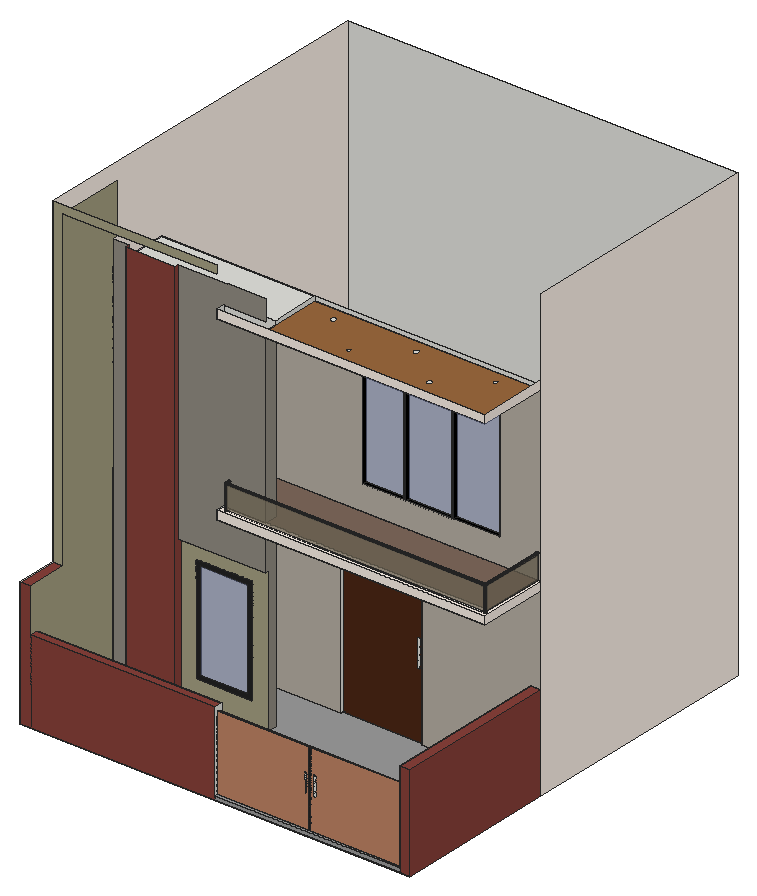
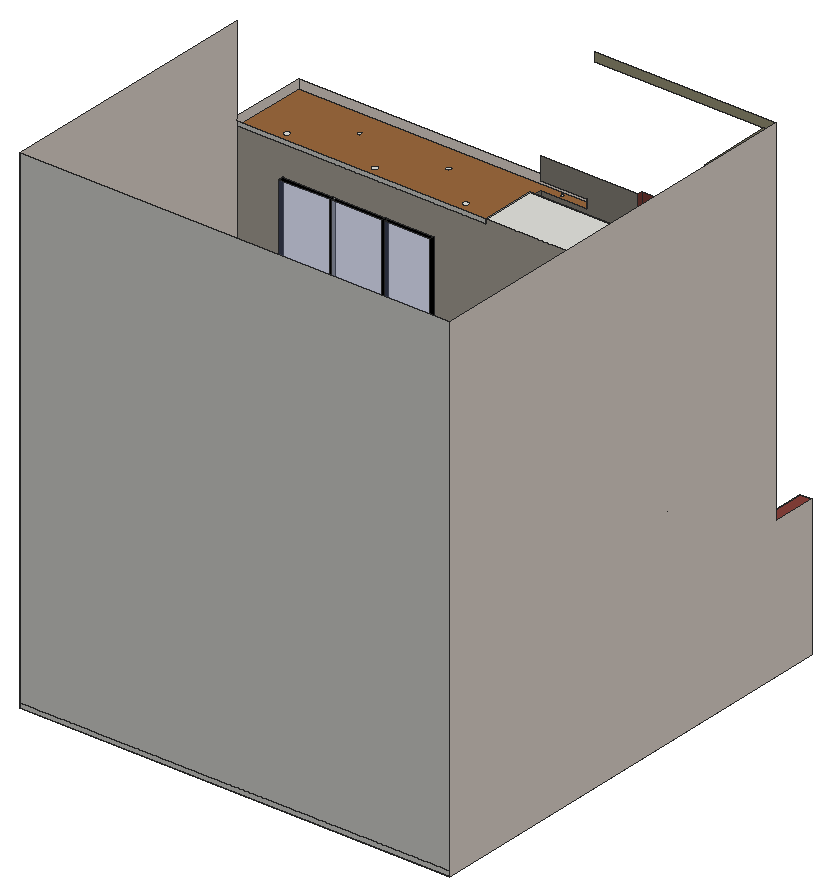
# SketchUp Ruby script. Lengths in inches.
U = 1.inch
M = Sketchup.active_model
def pt(a) = Geom::Point3d.new(a.map { |v| v * U })
def face(e, loops, mat)
  f = e.add_face(loops[0].map { |a| pt(a) })
  loops[1..].each { |l| e.add_face(l.map { |a| pt(a) }).erase! }
  f.material = f.back_material = mat if mat
  f
end
# faces: each face lists its corners as indices into pts; further lists are holes
def faces(e, pts, list, mat = nil) = list.each { |f| face(e, (f[0].is_a?(Array) ? f : [f]).map { |l| l.map { |i| pts[i] } }, mat) }
# xy, xz, yz: faces in a plane at the given z, y or x. An outline is a flat list of corners, or four numbers for a rectangle; further outlines are holes
def ring(l) = l.size == 4 ? [[l[0], l[1]], [l[2], l[1]], [l[2], l[3]], [l[0], l[3]]] : l.each_slice(2).to_a
def flat(e, list, mat, &to3) = list.each { |f| face(e, (f[0].is_a?(Array) ? f : [f]).map { |l| ring(l).map { |u, v| to3.(u, v) } }, mat) }
def xy(e, z, list, mat = nil) = flat(e, list, mat) { |x, y| [x, y, z] }
def xz(e, y, list, mat = nil) = flat(e, list, mat) { |x, z| [x, y, z] }
def yz(e, x, list, mat = nil) = flat(e, list, mat) { |y, z| [x, y, z] }
def lines(e, pts, list) = list.each { |a, b| e.add_line(pt(pts[a]), pt(pts[b])) }
# prism: a flat outline (further loops are holes) pulled along v
def prism(e, loops, v, mat = nil)
  f = face(e, loops, mat); d = Geom::Vector3d.new(v.map { |x| x * U })
  f.pushpull(f.normal.samedirection?(d) ? d.length : -d.length)
end
def box(e, o, s, mat = nil) = prism(e, [[o, [o[0] + s[0], o[1], o[2]], [o[0] + s[0], o[1] + s[1], o[2]], [o[0], o[1] + s[1], o[2]]]], [0, 0, s[2]], mat)
def at(x, y, z, deg = 0) = Geom::Transformation.translation(pt([x, y, z])) * Geom::Transformation.rotation(ORIGIN, Z_AXIS, deg.degrees)
def axes(o, x, y, z) = Geom::Transformation.new([*x, 0, *y, 0, *z, 0, *pt(o).to_a, 1])
def part(name) = M.definitions.add(name)
# library, detail: a bought-in or finely detailed component or shape, given as its bounding box
def library(name, o, s) = part(name).tap { |d| box(d.entities, o, s) }
def detail(e, o, s) = box(e.add_group.entities, o, s)
def put(e, d, t, mat = nil) = e.add_instance(d, t).tap { |i| i.material = mat if mat }
def group(e, t, mat = nil) = e.add_group.tap { |g| g.transformation = t; g.material = mat if mat }.entities
root = M.entities
M.materials.add("[0009_Linen]").color = [250, 240, 230]
M.materials.add("[0042_Sienna]").color = [76, 39, 21]
M.materials.add("[0118_Thistle]").color = [216, 191, 216]
M.materials.add("[0136_Charcoal]").color = [35, 35, 35]
M.materials.add("[0137_Black]").color = [0, 0, 0]
M.materials.add("[Brick Antique 01]").color = [135, 65, 58]
M.materials.add("[Carrera Marble]").color = [155, 155, 155]
M.materials.add("[Cinder Block]").color = [145, 140, 130]
M.materials.add("[Granite Brown]").color = [126, 104, 91]
M.materials.add("[Modern Siding]").color = [191, 132, 100]
M.materials.add("[Stone Coursed Rough]").color = [165, 160, 130]
M.materials.add("[Stone Masonry Multi]").color = [182, 175, 164]
M.materials.add("[Translucent Glass Gray]").color = [128, 118, 98]
M.materials["[Translucent Glass Gray]"].alpha = 0.5
M.materials.add("[Translucent Glass Sky Reflection]").color = [126, 138, 183]
M.materials["[Translucent Glass Sky Reflection]"].alpha = 0.52
M.materials.add("[Wood Floor]").color = [155, 105, 61]
xy(root,0,[[0,0,1142.5,480],[0,480,1142.5,1200]])
xy(root,12,[[571.25,7.56,1112.5,12],[78,288,78,300,30,300,30,335,480,335,480,312,221.625,312,221.625,288]])
xy(root,12,[[571.25,0,1112.5,7.56],[571.25,12,1112.5,12,1112.5,480,792.82,480,792.82,486,556.82,486,556.82,480,30,480,30,335,480,335,480,312,221.625,312,221.625,288,78,288,78,300,30,300,30,24,571.25,24]],"[Carrera Marble]")
xy(root,230.51,[[571.25,7.56,840.11,12],[840.11,7.56,847.05,12],[847.05,7.56,1112.5,12]],"[0136_Charcoal]")
xy(root,243.4375,[[30,0,571.25,24]],"[Brick Antique 01]")
xy(root,279.4375,[[1112.5,0,1142.5,480]],"[Brick Antique 01]")
xy(root,371.375,[[0,0,30,120]],"[Brick Antique 01]")
xy(root,408.875,[[556.82,480,792.82,486]])
xy(root,432,[[221.625,300,480,312]])
xy(root,540,[[427.52,280.89,425.97,281.09,424.52,281.69,423.28,282.64,422.32,283.89,421.72,285.33,421.52,286.89,421.72,288.4375,422.32,289.89,423.28,291.13,424.52,292.08,425.97,292.68,427.52,292.89,429.07,292.68,430.52,292.08,431.76,291.13,432.72,289.89,433.31,288.4375,433.52,286.89,433.31,285.33,432.72,283.89,431.76,282.64,430.52,281.69,429.07,281.09],[572.42,313.71,570.1,314.02,567.92,314.91,566.0625,316.35,564.63,318.21,563.73,320.38,563.42,322.71,563.73,325.04,564.63,327.21,566.0625,329.07,567.92,330.5,570.1,331.4,572.42,331.71,574.75,331.4,576.92,330.5,578.79,329.07,580.22,327.21,581.12,325.04,581.42,322.71,581.12,320.38,580.22,318.21,578.79,316.35,576.92,314.91,574.75,314.02],[783.17,313.71,780.85,314.02,778.67,314.91,776.8125,316.35,775.38,318.21,774.48,320.38,774.17,322.71,774.48,325.04,775.38,327.21,776.8125,329.07,778.67,330.5,780.85,331.4,783.17,331.71,785.5,331.4,787.67,330.5,789.54,329.07,790.97,327.21,791.87,325.04,792.17,322.71,791.87,320.38,790.97,318.21,789.54,316.35,787.67,314.91,785.5,314.02],[1004.8,313.71,1002.47,314.02,1000.3,314.91,998.4375,316.35,997.01,318.21,996.11,320.38,995.8,322.71,996.11,325.04,997.01,327.21,998.4375,329.07,1000.3,330.5,1002.47,331.4,1004.8,331.71,1007.13,331.4,1009.3,330.5,1011.16,329.07,1012.59,327.21,1013.49,325.04,1013.8,322.71,1013.49,320.38,1012.59,318.21,1011.16,316.35,1009.3,314.91,1007.13,314.02],[663.81,382.49,661.48,382.8,659.31,383.7,657.45,385.125,656.02,386.99,655.12,389.16,654.81,391.49,655.12,393.82,656.02,395.99,657.45,397.85,659.31,399.28,661.48,400.18,663.81,400.49,666.14,400.18,668.31,399.28,670.17,397.85,671.6,395.99,672.5,393.82,672.81,391.49,672.5,389.16,671.6,386.99,670.17,385.125,668.31,383.7,666.14,382.8],
  [918,382.49,915.67,382.8,913.5,383.7,911.63,385.125,910.2,386.99,909.3,389.16,909,391.49,909.3,393.82,910.2,395.99,911.63,397.85,913.5,399.28,915.67,400.18,918,400.49,920.33,400.18,922.5,399.28,924.36,397.85,925.79,395.99,926.69,393.82,927,391.49,926.69,389.16,925.79,386.99,924.36,385.125,922.5,383.7,920.33,382.8]])
xy(root,540,[[[355.9375,276,355.9375,300,480,300,480,480,1142.5,480,1142.5,276],[918,382.49,920.33,382.8,922.5,383.7,924.36,385.125,925.79,386.99,926.69,389.16,927,391.49,926.69,393.82,925.79,395.99,924.36,397.85,922.5,399.28,920.33,400.18,918,400.49,915.67,400.18,913.5,399.28,911.63,397.85,910.2,395.99,909.3,393.82,909,391.49,909.3,389.16,910.2,386.99,911.63,385.125,913.5,383.7,915.67,382.8],[663.81,382.49,666.14,382.8,668.31,383.7,670.17,385.125,671.6,386.99,672.5,389.16,672.81,391.49,672.5,393.82,671.6,395.99,670.17,397.85,668.31,399.28,666.14,400.18,663.81,400.49,661.48,400.18,659.31,399.28,657.45,397.85,656.02,395.99,655.12,393.82,654.81,391.49,655.12,389.16,656.02,386.99,657.45,385.125,659.31,383.7,661.48,382.8],[572.42,313.71,574.75,314.02,576.92,314.91,578.79,316.35,580.22,318.21,581.12,320.38,581.42,322.71,581.12,325.04,580.22,327.21,578.79,329.07,576.92,330.5,574.75,331.4,572.42,331.71,570.1,331.4,567.92,330.5,566.0625,329.07,564.63,327.21,563.73,325.04,563.42,322.71,563.73,320.38,564.63,318.21,566.0625,316.35,567.92,314.91,570.1,314.02],[783.17,313.71,785.5,314.02,787.67,314.91,789.54,316.35,790.97,318.21,791.87,320.38,792.17,322.71,791.87,325.04,790.97,327.21,789.54,329.07,787.67,330.5,785.5,331.4,783.17,331.71,780.85,331.4,778.67,330.5,776.8125,329.07,775.38,327.21,774.48,325.04,774.17,322.71,774.48,320.38,775.38,318.21,776.8125,316.35,778.67,314.91,780.85,314.02],[1004.8,313.71,1007.13,314.02,1009.3,314.91,1011.16,316.35,1012.59,318.21,1013.49,320.38,1013.8,322.71,1013.49,325.04,1012.59,327.21,1011.16,329.07,1009.3,330.5,1007.13,331.4,1004.8,331.71,1002.47,331.4,1000.3,330.5,998.4375,329.07,997.01,327.21,996.11,325.04,995.8,322.71,996.11,320.38,997.01,318.21,998.4375,316.35,1000.3,314.91,1002.47,314.02],[427.52,280.89,429.07,281.09,430.52,281.69,431.76,282.64,432.72,283.89,433.31,285.33,433.52,286.89,433.31,288.4375,432.72,289.89,431.76,291.13,430.52,292.08,429.07,292.68,427.52,292.89,425.97,292.68,424.52,292.08,423.28,291.13,422.32,289.89,421.72,288.4375,421.52,286.89,421.72,285.33,422.32,283.89,423.28,282.64,424.52,281.69,425.97,281.09]]],"[Wood Floor]")
xy(root,552,[[30,335,480,480]])
xy(root,564,[[372.86,284.19,372.1,284.36,371.4,284.71,370.82,285.24,370.4,285.9,370.16,286.64,370.12,287.43,370.28,288.19,370.64,288.89,371.17,289.47,371.82,289.89,372.57,290.13,373.35,290.17,374.12,290.01,374.81,289.65,375.39,289.12,375.82,288.46,375.97,288,375.97,286.34,375.93,286.17,375.57,285.47,375.05,284.89,374.39,284.47,373.64,284.23],[1133.61,284.19,1132.85,284.36,1132.15,284.71,1131.57,285.24,1131.15,285.9,1130.99,286.38,1130.99,288,1131.03,288.19,1131.39,288.89,1131.92,289.47,1132.57,289.89,1133.32,290.13,1133.5,290.14,1134.24,290.14,1134.87,290.01,1135.56,289.65,1136.14,289.12,1136.57,288.46,1136.81,287.72,1136.85,286.9375,1136.68,286.17,1136.32,285.47,1135.8,284.89,1135.14,284.47,1134.39,284.23],[375.97,286,375.97,286.34,376.1,286.9375,376.06,287.72,375.97,288,1124.5,288,1124.5,286],[1124.5,286,1124.5,288,1130.99,288,1130.87,287.43,1130.91,286.64,1130.99,286.38,1130.99,286],[375.97,286.34,375.97,288,376.06,287.72,376.1,286.9375],
  [1130.99,286.38,1130.91,286.64,1130.87,287.43,1130.99,288],[1124.5,288,1130.99,288,1131.03,288.19,1131.39,288.89,1131.92,289.47,1132.57,289.89,1133.32,290.13,1133.5,290.14,1133.5,300,1124.5,300],[1133.5,290.14,1133.5,300,1135.5,300,1135.5,290.14,1134.24,290.14,1134.1,290.17],[1133.5,290.14,1134.1,290.17,1134.24,290.14],[1133.5,300,1135.5,480]])
xy(root,564,[[355.9375,276,1142.5,276,1142.5,480,1135.5,480,1135.5,290.14,1134.24,290.14,1134.87,290.01,1135.56,289.65,1136.14,289.12,1136.57,288.46,1136.81,287.72,1136.85,286.9375,1136.68,286.17,1136.32,285.47,1135.8,284.89,1135.14,284.47,1134.39,284.23,1133.61,284.19,1132.85,284.36,1132.15,284.71,1131.57,285.24,1131.15,285.9,1130.99,286.38,1130.99,286,375.97,286,375.97,286.34,375.93,286.17,375.57,285.47,375.05,284.89,374.39,284.47,373.64,284.23,372.86,284.19,372.1,284.36,371.4,284.71,370.82,285.24,370.4,285.9,370.16,286.64,370.12,287.43,370.28,288.19,370.64,288.89,371.17,289.47,371.82,289.89,372.57,290.13,373.35,290.17,374.12,290.01,374.81,289.65,375.39,289.12,375.82,288.46,375.97,288,1124.5,288,1124.5,300,355.9375,300]],"[0009_Linen]")
xy(root,564,[[480,300,1133.5,300,1133.5,480,30,480,30,335,480,335]],"[Granite Brown]")
xy(root,632,[[1133.5,290.14,1135.5,480]])
xy(root,632.1875,[[375.97,286,376.01,288],[376.01,286,376.04,288],[376.04,286,1130.99,288]])
xy(root,637.48,[[619.18,480,740.94,492],[746.94,480,881.44,492],[887.44,480,1021.8,492]],"[0137_Black]")
xy(root,989.04,[[619.18,480,740.94,492],[746.94,480,881.44,492],[887.44,480,1021.8,492]],"[0137_Black]")
xy(root,1068,[[431.18,281.55,429.63,281.76,428.18,282.36,426.9375,283.31,425.98,284.55,425.39,286,425.18,287.55,425.39,289.11,425.98,290.55,426.9375,291.8,428.18,292.75,429.63,293.35,431.18,293.55,432.73,293.35,434.18,292.75,435.42,291.8,436.375,290.55,436.98,289.11,437.18,287.55,436.98,286,436.375,284.55,435.42,283.31,434.18,282.36,432.73,281.76],[686.16,340.72,684.6,340.87,683.13,341.42,681.86,342.33,680.86,343.53,680.21,344.96,679.95,346.5,680.1,348.0625,680.64,349.53,681.55,350.81,682.76,351.8,684.1875,352.45,685.73,352.71,687.29,352.57,688.76,352.02,690.03,351.11,691.03,349.9,691.68,348.48,691.94,346.93,691.79,345.375,691.25,343.91,690.34,342.63,689.13,341.63,687.7,340.98],[923.28,340.72,921.73,340.87,920.26,341.42,918.98,342.33,917.98,343.53,917.33,344.96,917.07,346.5,917.22,348.0625,917.77,349.53,918.68,350.81,919.89,351.8,921.3125,352.45,922.86,352.71,924.41,352.57,925.88,352.02,927.16,351.11,928.16,349.9,928.81,348.48,929.07,346.93,928.92,345.375,928.37,343.91,927.46,342.63,926.25,341.63,924.83,340.98],[567.52,433.08,565.96,433.23,564.49,433.78,563.21,434.68,562.22,435.89,561.57,437.32,561.31,438.86,561.45,440.42,562,441.89,562.91,443.16,564.12,444.16,565.54,444.8125,567.09,445.07,568.65,444.92,570.11,444.375,571.39,443.47,572.39,442.26,573.04,440.84,573.3,439.29,573.15,437.73,572.6,436.26,571.69,434.99,570.49,433.99,569.0625,433.34],[809.39,433.08,807.83,433.23,806.36,433.78,805.09,434.68,804.09,435.89,803.44,437.32,803.18,438.86,803.33,440.42,803.875,441.89,804.78,443.16,805.99,444.16,807.42,444.8125,808.96,445.07,810.52,444.92,811.99,444.375,813.26,443.47,814.26,442.26,814.91,440.84,815.17,439.29,815.02,437.73,814.48,436.26,813.57,434.99,812.36,433.99,810.9375,433.34],
  [1042.39,433.08,1040.83,433.23,1039.36,433.78,1038.09,434.68,1037.09,435.89,1036.44,437.32,1036.18,438.86,1036.33,440.42,1036.875,441.89,1037.78,443.16,1038.99,444.16,1040.42,444.8125,1041.96,445.07,1043.52,444.92,1044.99,444.375,1046.26,443.47,1047.26,442.26,1047.91,440.84,1048.17,439.29,1048.02,437.73,1047.48,436.26,1046.57,434.99,1045.36,433.99,1043.9375,433.34]])
xy(root,1068,[[[355.9375,276,355.9375,300,480,300,480,480,1142.5,480,1142.5,276],[431.18,281.55,432.73,281.76,434.18,282.36,435.42,283.31,436.375,284.55,436.98,286,437.18,287.55,436.98,289.11,436.375,290.55,435.42,291.8,434.18,292.75,432.73,293.35,431.18,293.55,429.63,293.35,428.18,292.75,426.9375,291.8,425.98,290.55,425.39,289.11,425.18,287.55,425.39,286,425.98,284.55,426.9375,283.31,428.18,282.36,429.63,281.76],[567.52,433.08,569.0625,433.34,570.49,433.99,571.69,434.99,572.6,436.26,573.15,437.73,573.3,439.29,573.04,440.84,572.39,442.26,571.39,443.47,570.11,444.375,568.65,444.92,567.09,445.07,565.54,444.8125,564.12,444.16,562.91,443.16,562,441.89,561.45,440.42,561.31,438.86,561.57,437.32,562.22,435.89,563.21,434.68,564.49,433.78,565.96,433.23],[1042.39,433.08,1043.9375,433.34,1045.36,433.99,1046.57,434.99,1047.48,436.26,1048.02,437.73,1048.17,439.29,1047.91,440.84,1047.26,442.26,1046.26,443.47,1044.99,444.375,1043.52,444.92,1041.96,445.07,1040.42,444.8125,1038.99,444.16,1037.78,443.16,1036.875,441.89,1036.33,440.42,1036.18,438.86,1036.44,437.32,1037.09,435.89,1038.09,434.68,1039.36,433.78,1040.83,433.23],[809.39,433.08,810.9375,433.34,812.36,433.99,813.57,434.99,814.48,436.26,815.02,437.73,815.17,439.29,814.91,440.84,814.26,442.26,813.26,443.47,811.99,444.375,810.52,444.92,808.96,445.07,807.42,444.8125,805.99,444.16,804.78,443.16,803.875,441.89,803.33,440.42,803.18,438.86,803.44,437.32,804.09,435.89,805.09,434.68,806.36,433.78,807.83,433.23],[686.16,340.72,687.7,340.98,689.13,341.63,690.34,342.63,691.25,343.91,691.79,345.375,691.94,346.93,691.68,348.48,691.03,349.9,690.03,351.11,688.76,352.02,687.29,352.57,685.73,352.71,684.1875,352.45,682.76,351.8,681.55,350.81,680.64,349.53,680.1,348.0625,679.95,346.5,680.21,344.96,680.86,343.53,681.86,342.33,683.13,341.42,684.6,340.87],[923.28,340.72,924.83,340.98,926.25,341.63,927.46,342.63,928.37,343.91,928.92,345.375,929.07,346.93,928.81,348.48,928.16,349.9,927.16,351.11,925.88,352.02,924.41,352.57,922.86,352.71,921.3125,352.45,919.89,351.8,918.68,350.81,917.77,349.53,917.22,348.0625,917.07,346.5,917.33,344.96,917.98,343.53,918.98,342.33,920.26,341.42,921.73,340.87]]],"[Wood Floor]")
xy(root,1080,[[30,335,480,480]])
xz(root,0,[[0,0,30,371.375],[30,0,571.25,243.4375],[1112.5,0,1142.5,279.4375]],"[Brick Antique 01]")
xz(root,0,[[571.25,0,1112.5,12]],"[Carrera Marble]")
xz(root,7.56,[[827.63,104.83,833.57,161.14],[853.32,104.83,859.25,161.14]])
xz(root,7.56,[[840.11,12,847.05,230.51]],"[0136_Charcoal]")
xz(root,7.56,[[[571.25,12,840.11,230.51],[827.63,104.83,833.57,161.14]],[[847.05,12,1112.5,230.51],[853.32,104.83,859.25,161.14]]],"[Modern Siding]")
xz(root,12,[[840.11,12,847.05,230.51]])
xz(root,12,[[571.25,12,840.11,230.51],[847.05,12,1112.5,230.51]],"[Modern Siding]")
xz(root,24,[[30,12,571.25,243.4375]],"[Brick Antique 01]")
xz(root,120,[[0,371.375,30,371.375,30,1296,480,1296,480,1320,0,1320]],"[Stone Coursed Rough]")
xz(root,276,[[355.9375,540,1142.5,564],[355.9375,1068,1142.5,1092]],"[0009_Linen]")
xz(root,286,[[375.97,564,1130.99,632.1875]],"[Translucent Glass Gray]")
xz(root,288,[[78,12,221.625,1152]],"[Brick Antique 01]")
xz(root,288,[[375.97,564,1130.99,632.1875]],"[Translucent Glass Gray]")
xz(root,290.14,[[1133.5,564,1135.5,630],[1133.5,630,1135.5,632]])
xz(root,290.16,[[1133.86,633,1134.63,633.1,1135.36,633.4,1135.98,633.88,1136.46,634.5,1136.76,635.22,1136.86,636,1136.76,636.78,1136.46,637.5,1135.98,638.12,1135.36,638.6,1134.63,638.9,1133.86,639,1133.08,638.9,1132.36,638.6,1131.74,638.12,1131.26,637.5,1130.96,636.78,1130.86,636,1130.96,635.22,1131.26,634.5,1131.74,633.88,1132.36,633.4,1133.08,633.1]])
xz(root,300,[[355.9375,540,480,564]])
xz(root,300,[[30,12,78,1152],[[221.625,432,480,432,480,540,355.9375,540,355.9375,564,480,564,480,1068,355.9375,1068,355.9375,1092,480,1092,480,1152,370.55,1152,370.44,1151.22,370.14,1150.5,369.67,1149.88,369.05,1149.4,368.32,1149.1,367.55,1149,366.77,1149.1,366.05,1149.4,365.43,1149.88,364.95,1150.5,364.65,1151.22,364.55,1152,221.625,1152],[373.35,633.01,372.57,633.05,371.82,633.29,371.17,633.71,370.64,634.29,370.28,634.99,370.12,635.75,370.16,636.54,370.4,637.28,370.82,637.94,371.4,638.47,372.1,638.82,372.86,638.99,373.64,638.95,374.39,638.71,375.05,638.29,375.57,637.71,375.93,637.01,376.1,636.25,376.06,635.46,375.82,634.72,375.39,634.06,374.81,633.53,374.12,633.18]]],"[Cinder Block]")
xz(root,312,[[[264.98,72.93,432.66,389.18],[279.75,87.7,417.89,374.41]]],"[0136_Charcoal]")
xz(root,312,[[[221.625,12,480,432],[264.98,72.93,432.66,389.18]]],"[Stone Coursed Rough]")
xz(root,312,[[279.75,87.7,417.89,374.41]],"[Translucent Glass Sky Reflection]")
xz(root,335,[[30,12,480,552],[30,564,480,1080]])
xz(root,480,[[1112.5,12,1142.5,279.4375],[480,540,1142.5,552],[480,552,1142.5,564],[1133.5,564,1135.5,632],[1133.86,633,1133.08,633.1,1132.36,633.4,1131.74,633.88,1131.26,634.5,1130.96,635.22,1130.86,636,1130.96,636.78,1131.26,637.5,1131.74,638.12,1132.36,638.6,1133.08,638.9,1133.86,639,1134.63,638.9,1135.36,638.6,1135.98,638.12,1136.46,637.5,1136.76,636.78,1136.86,636,1136.76,635.22,1136.46,634.5,1135.98,633.88,1135.36,633.4,1134.63,633.1],
  [480,1068,1142.5,1080]])
xz(root,480,[[740.94,637.48,746.94,989.04],[881.44,637.48,887.44,989.04]],"[0137_Black]")
xz(root,480,[[30,12,556.82,12,556.82,408.875,792.82,408.875,792.82,12,1112.5,12,1112.5,279.4375,1142.5,279.4375,1142.5,540,480,540,480,552,30,552],[[30,564,1133.5,564,1133.5,632,1135.5,632,1135.5,564,1142.5,564,1142.5,1068,480,1068,480,1080,30,1080],[619.18,637.48,1021.8,989.04],[1133.86,633,1133.08,633.1,1132.36,633.4,1131.74,633.88,1131.26,634.5,1130.96,635.22,1130.86,636,1130.96,636.78,1131.26,637.5,1131.74,638.12,1132.36,638.6,1133.08,638.9,1133.86,639,1134.63,638.9,1135.36,638.6,1135.98,638.12,1136.46,637.5,1136.76,636.78,1136.86,636,1136.76,635.22,1136.46,634.5,1135.98,633.88,1135.36,633.4,1134.63,633.1]]],"[Stone Masonry Multi]")
xz(root,486,[[556.82,12,792.82,12.5],[777.65,205.33,782.4,285.39]])
xz(root,486,[[[556.82,12.5,792.82,408.875],[777.65,205.33,782.4,285.39]]],"[0042_Sienna]")
xz(root,492,[[619.18,637.48,740.94,989.04],[746.94,637.48,881.44,989.04],[887.44,637.48,1021.8,989.04]],"[Translucent Glass Sky Reflection]")
xz(root,1200,[[0,0,1142.5,12],[0,12,1142.5,1320]])
yz(root,0,[[0,0,0,371.375,120,371.375,120,1320,1200,1320,1200,0]],"[0009_Linen]")
yz(root,30,[[300,12,335,552],[300,564,335,1080]])
yz(root,30,[[335,12,480,552],[335,564,480,1080]],"[0118_Thistle]")
yz(root,30,[[24,12,300,12,300,1152,318,1152,318,1296,120,1296,120,371.375,0,371.375,0,243.4375,24,243.4375]],"[Stone Coursed Rough]")
yz(root,78,[[288,12,300,1152]],"[Brick Antique 01]")
yz(root,221.625,[[288,12,312,12,312,432,300,432,300,1152,288,1152]],"[Brick Antique 01]")
yz(root,355.9375,[[276,540,300,564],[276,1068,300,1092]])
yz(root,375.97,[[286,564,288,632],[286,632,288,632.1875]])
yz(root,376.09,[[287.43,633.01,286.64,633.05,285.9,633.29,285.24,633.71,284.71,634.29,284.36,634.99,284.19,635.75,284.23,636.54,284.47,637.28,284.89,637.94,285.47,638.47,286.17,638.82,286.9375,638.99,287.72,638.95,288.46,638.71,289.12,638.29,289.65,637.71,290.01,637.01,290.17,636.25,290.13,635.46,289.89,634.72,289.47,634.06,288.89,633.53,288.19,633.18]])
yz(root,480,[[335,540,480,552],[335,1068,480,1080]])
yz(root,480,[[312,12,335,12,335,540,300,540,300,432,312,432],[300,564,335,1068]],"[Cinder Block]")
yz(root,556.82,[[480,12,486,12.5],[480,12.5,486,408.875]])
yz(root,571.25,[[0,12,7.56,12,7.56,230.51,12,230.51,12,12,24,12,24,243.4375,0,243.4375],[7.56,12,12,230.51]])
yz(root,619.18,[[480,637.48,492,989.04]],"[0137_Black]")
yz(root,740.94,[[480,637.48,492,989.04]],"[0137_Black]")
yz(root,746.94,[[480,637.48,492,989.04]],"[0137_Black]")
yz(root,792.82,[[480,12,486,12.5],[480,12.5,486,408.875]])
yz(root,881.44,[[480,637.48,492,989.04]])
yz(root,887.44,[[480,637.48,492,989.04]],"[0137_Black]")
yz(root,1021.8,[[480,637.48,492,989.04]],"[0137_Black]")
yz(root,1112.5,[[0,12,0,279.4375,480,279.4375,480,12,12,12,12,230.51,7.56,230.51,7.56,12]],"[Brick Antique 01]")
yz(root,1130.99,[[286,564,288,630],[286,630,288,632.1875]])
yz(root,1133.5,[[290.14,564,480,632]],"[Translucent Glass Gray]")
yz(root,1135.5,[[290.14,564,480,632]],"[Translucent Glass Gray]")
yz(root,1142.5,[[480,0,1200,1320],[276,540,480,564],[276,1068,480,1092]],"[0009_Linen]")
yz(root,1142.5,[[0,0,480,279.4375]],"[Brick Antique 01]")
p = [[372.1,284.36,564],[372.86,284.19,564],[372.86,284.19,638.99],[372.1,284.36,638.82],[373.64,284.23,564],[373.64,284.23,638.95],
  [374.39,284.47,564],[374.39,284.47,638.71],[1132.85,284.36,564],[1133.61,284.19,564],[1133.61,284.19,635.75],[1132.85,284.36,634.99],
  [1134.39,284.23,564],[1134.39,284.23,636.54],[1135.14,284.47,564],[1135.14,284.47,637.28],[371.4,284.71,564],[371.4,284.71,638.47],
  [1132.15,284.71,564],[1132.15,284.71,634.29],[375.05,284.89,564],[375.05,284.89,638.29],[1135.8,284.89,564],[1135.8,284.89,637.94],
  [370.82,285.24,564],[370.82,285.24,637.94],[1131.57,285.24,564],[1131.57,285.24,633.71],[375.57,285.47,564],[375.57,285.47,637.71],
  [1136.32,285.47,564],[1136.32,285.47,638.47],[370.4,285.9,564],[370.4,285.9,637.28],[1131.15,285.9,564],[1131.15,285.9,633.29],
  [375.93,286.17,564],[375.93,286.17,637.01],[1136.68,286.17,564],[1136.68,286.17,638.82],[370.16,286.64,564],[370.16,286.64,636.54],
  [1130.91,286.64,564],[1130.99,286.38,564],[1130.91,286.64,633.05],[375.97,286.34,564],[376.1,286.9375,564],[376.1,286.9375,636.25],
  [1136.85,286.9375,564],[1136.85,286.9375,638.99],[370.12,287.43,564],[370.12,287.43,635.75],[1130.87,287.43,564],[1130.87,287.43,633.01],
  [376.06,287.72,564],[376.06,287.72,635.46],[376.09,287.18,636],[1136.81,287.72,564],[1136.81,287.72,638.95],[370.28,288.19,564],
  [370.28,288.19,634.99],[1131.03,288.19,564],[1130.99,288,564],[1131.03,288.19,633.18],[375.97,288,564],[375.82,288.46,564],
  [375.82,288.46,634.72],[1136.57,288.46,564],[1136.57,288.46,638.71],[370.64,288.89,564],[370.64,288.89,634.29],[1131.39,288.89,564],
  [1131.39,288.89,633.53],[375.39,289.12,564],[375.39,289.12,634.06],[1136.14,289.12,564],[1136.14,289.12,638.29],[371.17,289.47,564],
  [371.17,289.47,633.71],[1131.92,289.47,564],[1131.92,289.47,634.06],[374.81,289.65,564],[374.81,289.65,633.53],[1135.56,289.65,564],
  [1135.56,289.65,637.71],[371.82,289.89,564],[371.82,289.89,633.29],[1132.57,289.89,564],[1132.57,289.89,634.72],[374.12,290.01,564],
  [374.12,290.01,633.18],[1134.87,290.01,564],[1134.87,290.01,637.01],[372.57,290.13,564],[372.57,290.13,633.05],[1133.32,290.13,564],
  [1133.32,290.13,635.46],[373.35,290.17,564],[373.35,290.17,633.01],[1134.24,290.14,564],[1134.1,290.17,564],[1134.1,290.17,636.25],
  [1133.5,290.14,564],[1133.86,290.16,636],[376.09,285.9,633.29],[376.09,286.64,633.05],[376.09,287.43,633.01],[376.09,288.19,633.18],
  [371.82,300,633.29],[372.57,300,633.05],[373.35,300,633.01],[374.12,300,633.18],[1133.08,480,633.1],[1133.86,480,633],
  [1133.86,290.16,633],[1133.08,290.16,633.1],[1134.63,480,633.1],[1134.63,290.16,633.1],[1132.36,480,633.4],[1132.36,290.16,633.4],
  [1135.36,480,633.4],[1135.36,290.16,633.4],[376.09,288.89,633.53],[374.81,300,633.53],[376.09,285.24,633.71],[371.17,300,633.71],
  [1131.74,480,633.88],[1131.74,290.16,633.88],[1135.98,480,633.88],[1135.98,290.16,633.88],[376.09,289.47,634.06],[375.39,300,634.06],
  [376.09,284.71,634.29],[370.64,300,634.29],[1131.26,480,634.5],[1131.26,290.16,634.5],[1136.46,480,634.5],[1136.46,290.16,634.5],
  [375.82,300,634.72],[376.09,289.89,634.72],[376.09,284.36,634.99],[370.28,300,634.99],[1130.96,480,635.22],[1130.96,290.16,635.22],
  [1136.76,480,635.22],[1136.76,290.16,635.22],[376.06,300,635.46],[376.09,290.13,635.46],[376.09,284.19,635.75],[370.12,300,635.75],
  [1130.86,480,636],[1130.86,290.16,636],[1136.86,480,636],[1136.86,290.16,636],[376.1,300,636.25],[376.1,290.17,636.25],
  [376.09,290.17,636.25],[376.09,284.23,636.54],[370.16,300,636.54],[1130.96,480,636.78],[1130.96,290.16,636.78],[1136.76,480,636.78],
  [1136.76,290.16,636.78],[375.93,300,637.01],[376.09,290.01,637.01],[376.09,284.47,637.28],[370.4,300,637.28],[1131.26,480,637.5],
  [1131.26,290.16,637.5],[1136.46,480,637.5],[1136.46,290.16,637.5],[375.57,300,637.71],[376.09,289.65,637.71],[376.09,284.89,637.94],
  [370.82,300,637.94],[1131.74,480,638.12],[1131.74,290.16,638.12],[1135.98,480,638.12],[1135.98,290.16,638.12],[375.05,300,638.29],
  [376.09,289.12,638.29],[371.4,300,638.47],[376.09,285.47,638.47],[1132.36,480,638.6],[1132.36,290.16,638.6],[1135.36,480,638.6],
  [1135.36,290.16,638.6],[374.39,300,638.71],[376.09,288.46,638.71],[372.1,300,638.82],[376.09,286.17,638.82],[1133.08,480,638.9],
  [1133.08,290.16,638.9],[1134.63,480,638.9],[1134.63,290.16,638.9],[373.64,300,638.95],[376.09,287.72,638.95],[372.86,300,638.99],
  [376.09,286.9375,638.99],[1133.86,480,639],[1133.86,290.16,639],[0,480,552],[30,480,552],[1133.86,287.18,564],
  [1133.86,287.18,636],[373.11,287.18,564],[373.11,287.18,636],[373.11,300,636],[1133.86,480,636]]
faces(root,p,[[0,1,2,3],[1,4,5,2],[4,6,7,5],[8,9,10,11],[9,12,13,10],[12,14,15,13],[16,0,3,17],[18,8,11,19],
  [6,20,21,7],[14,22,23,15],[24,16,17,25],[26,18,19,27],[20,28,29,21],[22,30,31,23],[32,24,25,33],[34,26,27,35],
  [28,36,37,29],[30,38,39,31],[40,32,33,41],[42,43,34,35,44],[36,45,46,47,37],[38,48,49,39],[50,40,41,51],[52,42,44,53],
  [46,54,55,56,47],[48,57,58,49],[59,50,51,60],[61,62,52,53,63],[54,64,65,66,55],[57,67,68,58],[69,59,60,70],[71,61,63,72],
  [65,73,74,66],[67,75,76,68],[77,69,70,78],[79,71,72,80],[73,81,82,74],[75,83,84,76],[85,77,78,86],[87,79,80,88],
  [81,89,90,82],[83,91,92,84],[93,85,86,94],[95,87,88,96],[89,97,98,90],[91,99,100,101,92],[97,93,94,98],[100,102,95,96,103,101],
  [44,35,104,105],[53,44,105,106],[63,53,106,107],[94,86,108,109],[90,98,110,111],[98,94,109,110],[112,113,114,115],[113,116,117,114],
  [118,112,115,119],[116,120,121,117],[72,63,107,122],[82,90,111,123],[35,27,124,104],[86,78,125,108],[126,118,119,127],[120,128,129,121],
  [80,72,122,130],[74,82,123,131],[27,19,132,124],[78,70,133,125],[134,126,127,135],[128,136,137,129],[66,74,131,138],[88,80,130,139],
  [19,11,140,132],[70,60,141,133],[142,134,135,143],[136,144,145,137],[55,66,138,146],[96,88,139,147],[11,10,148,140],[60,51,149,141],
  [150,142,143,151],[144,152,153,145],[56,55,146,154,155,47],[103,96,147,156,155,101],[10,13,157,148],[51,41,158,149],[159,150,151,160],[152,161,162,153],
  [37,47,155,154,163],[92,101,155,156,164],[13,15,165,157],[41,33,166,158],[167,159,160,168],[161,169,170,162],[29,37,163,171],[84,92,164,172],
  [15,23,173,165],[33,25,174,166],[175,167,168,176],[169,177,178,170],[21,29,171,179],[76,84,172,180],[25,17,181,174],[23,31,182,173],
  [183,175,176,184],[177,185,186,178],[7,21,179,187],[68,76,180,188],[17,3,189,181],[31,39,190,182],[191,183,184,192],[185,193,194,186],
  [5,7,187,195],[58,68,188,196],[3,2,197,189],[39,49,198,190],[199,191,192,200],[193,199,200,194],[2,5,195,197],[49,58,196,198]])
lines(root,p,[[201,202],[203,204],[204,103],[205,206],[206,56],[206,207],[56,204],[103,208]])
